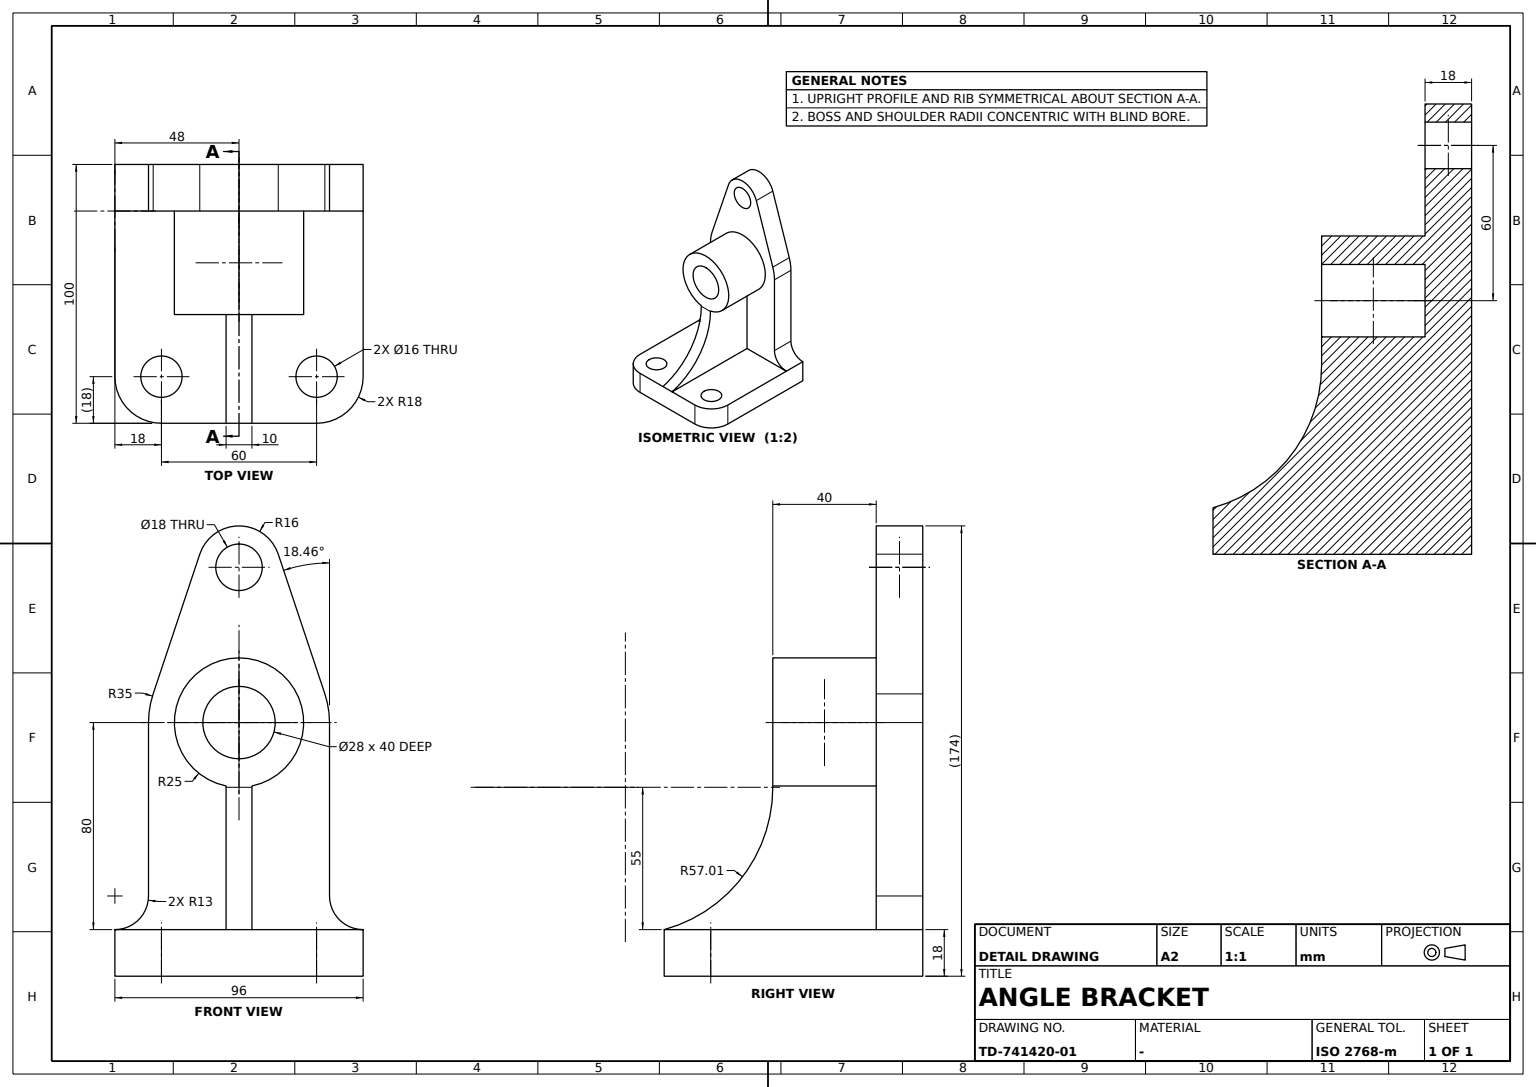
ISO-10303-21;
HEADER;
FILE_DESCRIPTION((''),'2;1');
FILE_NAME('','',(''),(''),'','','');
FILE_SCHEMA(('AUTOMOTIVE_DESIGN'));
ENDSEC;
DATA;
#1=APPLICATION_CONTEXT('');
#2=PRODUCT_CONTEXT('',#1,'mechanical');
#3=PRODUCT('','','',(#2));
#4=PRODUCT_DEFINITION_FORMATION('','',#3);
#5=PRODUCT_DEFINITION_CONTEXT('',#1,'design');
#6=PRODUCT_DEFINITION('','',#4,#5);
#7=PRODUCT_DEFINITION_SHAPE('','',#6);
#8=(LENGTH_UNIT()NAMED_UNIT(*)SI_UNIT(.MILLI.,.METRE.));
#9=(NAMED_UNIT(*)PLANE_ANGLE_UNIT()SI_UNIT($,.RADIAN.));
#10=(NAMED_UNIT(*)SI_UNIT($,.STERADIAN.)SOLID_ANGLE_UNIT());
#11=UNCERTAINTY_MEASURE_WITH_UNIT(LENGTH_MEASURE(0.005),#8,'distance_accuracy_value','');
#12=(GEOMETRIC_REPRESENTATION_CONTEXT(3)GLOBAL_UNCERTAINTY_ASSIGNED_CONTEXT((#11))GLOBAL_UNIT_ASSIGNED_CONTEXT((#8,#9,#10))REPRESENTATION_CONTEXT('',''));
#13=CARTESIAN_POINT('',(-48.,82.,0.));
#14=VERTEX_POINT('',#13);
#15=CARTESIAN_POINT('',(-48.,82.,-18.));
#16=VERTEX_POINT('',#15);
#17=CARTESIAN_POINT('',(-48.,82.,-9.));
#18=DIRECTION('',(0.,0.,1.));
#19=VECTOR('',#18,1000.);
#20=LINE('',#17,#19);
#21=EDGE_CURVE('',#14,#16,#20,.F.);
#22=ORIENTED_EDGE('',*,*,#21,.F.);
#23=CARTESIAN_POINT('',(-30.,100.,0.));
#24=VERTEX_POINT('',#23);
#25=CARTESIAN_POINT('',(-30.,82.,0.));
#26=DIRECTION('',(1.,0.,0.));
#27=AXIS2_PLACEMENT_3D('',#25,#18,#26);
#28=CIRCLE('',#27,18.);
#29=EDGE_CURVE('',#24,#14,#28,.T.);
#30=ORIENTED_EDGE('',*,*,#29,.F.);
#31=CARTESIAN_POINT('',(-30.,100.,-18.));
#32=VERTEX_POINT('',#31);
#33=CARTESIAN_POINT('',(-30.,100.,-9.));
#34=LINE('',#33,#19);
#35=EDGE_CURVE('',#24,#32,#34,.F.);
#36=ORIENTED_EDGE('',*,*,#35,.T.);
#37=CARTESIAN_POINT('',(-30.,82.,-18.));
#38=AXIS2_PLACEMENT_3D('',#37,#18,#26);
#39=CIRCLE('',#38,18.);
#40=EDGE_CURVE('',#32,#16,#39,.T.);
#41=ORIENTED_EDGE('',*,*,#40,.T.);
#42=EDGE_LOOP('',(#22,#30,#36,#41));
#43=FACE_BOUND('',#42,.T.);
#44=CARTESIAN_POINT('',(-30.,82.,-9.));
#45=AXIS2_PLACEMENT_3D('',#44,#18,#26);
#46=CYLINDRICAL_SURFACE('',#45,18.);
#47=ADVANCED_FACE('',(#43),#46,.T.);
#48=CARTESIAN_POINT('',(-35.,0.,80.));
#49=VERTEX_POINT('',#48);
#50=CARTESIAN_POINT('',(-33.198791,0.,91.083333));
#51=VERTEX_POINT('',#50);
#52=CARTESIAN_POINT('',(0.,0.,80.));
#53=DIRECTION('',(0.,-1.,0.));
#54=DIRECTION('',(0.,0.,-1.));
#55=AXIS2_PLACEMENT_3D('',#52,#53,#54);
#56=CIRCLE('',#55,35.);
#57=EDGE_CURVE('',#49,#51,#56,.F.);
#58=ORIENTED_EDGE('',*,*,#57,.T.);
#59=CARTESIAN_POINT('',(-33.198791,18.,91.083333));
#60=VERTEX_POINT('',#59);
#61=CARTESIAN_POINT('',(-33.198791,9.,91.083333));
#62=DIRECTION('',(0.,1.,0.));
#63=VECTOR('',#62,1000.);
#64=LINE('',#61,#63);
#65=EDGE_CURVE('',#51,#60,#64,.T.);
#66=ORIENTED_EDGE('',*,*,#65,.T.);
#67=CARTESIAN_POINT('',(-35.,18.,80.));
#68=VERTEX_POINT('',#67);
#69=CARTESIAN_POINT('',(0.,18.,80.));
#70=AXIS2_PLACEMENT_3D('',#69,#62,#18);
#71=CIRCLE('',#70,35.);
#72=EDGE_CURVE('',#68,#60,#71,.T.);
#73=ORIENTED_EDGE('',*,*,#72,.F.);
#74=CARTESIAN_POINT('',(-35.,9.,80.));
#75=LINE('',#74,#63);
#76=EDGE_CURVE('',#49,#68,#75,.T.);
#77=ORIENTED_EDGE('',*,*,#76,.F.);
#78=EDGE_LOOP('',(#58,#66,#73,#77));
#79=FACE_BOUND('',#78,.T.);
#80=CARTESIAN_POINT('',(0.,9.,80.));
#81=DIRECTION('',(-1.,0.,0.));
#82=AXIS2_PLACEMENT_3D('',#80,#62,#81);
#83=CYLINDRICAL_SURFACE('',#82,35.);
#84=ADVANCED_FACE('',(#79),#83,.T.);
#85=CARTESIAN_POINT('',(35.,18.,80.));
#86=VERTEX_POINT('',#85);
#87=CARTESIAN_POINT('',(35.,18.,13.));
#88=VERTEX_POINT('',#87);
#89=CARTESIAN_POINT('',(35.,18.,0.));
#90=VECTOR('',#54,1000.);
#91=LINE('',#89,#90);
#92=EDGE_CURVE('',#86,#88,#91,.T.);
#93=ORIENTED_EDGE('',*,*,#92,.F.);
#94=CARTESIAN_POINT('',(35.,0.,80.));
#95=VERTEX_POINT('',#94);
#96=CARTESIAN_POINT('',(35.,9.,80.));
#97=LINE('',#96,#63);
#98=EDGE_CURVE('',#95,#86,#97,.T.);
#99=ORIENTED_EDGE('',*,*,#98,.F.);
#100=CARTESIAN_POINT('',(35.,0.,13.));
#101=VERTEX_POINT('',#100);
#102=LINE('',#94,#90);
#103=EDGE_CURVE('',#95,#101,#102,.T.);
#104=ORIENTED_EDGE('',*,*,#103,.T.);
#105=CARTESIAN_POINT('',(35.,50.,13.));
#106=LINE('',#105,#63);
#107=EDGE_CURVE('',#101,#88,#106,.T.);
#108=ORIENTED_EDGE('',*,*,#107,.T.);
#109=EDGE_LOOP('',(#93,#99,#104,#108));
#110=FACE_BOUND('',#109,.T.);
#111=AXIS2_PLACEMENT_3D('',#94,#26,#54);
#112=PLANE('',#111);
#113=ADVANCED_FACE('',(#110),#112,.T.);
#114=CARTESIAN_POINT('',(-5.,100.,0.));
#115=VERTEX_POINT('',#114);
#116=CARTESIAN_POINT('',(5.,100.,0.));
#117=VERTEX_POINT('',#116);
#118=VECTOR('',#26,1000.);
#119=LINE('',#114,#118);
#120=EDGE_CURVE('',#115,#117,#119,.T.);
#121=ORIENTED_EDGE('',*,*,#120,.T.);
#122=CARTESIAN_POINT('',(30.,100.,0.));
#123=VERTEX_POINT('',#122);
#124=LINE('',#23,#118);
#125=EDGE_CURVE('',#117,#123,#124,.T.);
#126=ORIENTED_EDGE('',*,*,#125,.T.);
#127=CARTESIAN_POINT('',(30.,100.,-18.));
#128=VERTEX_POINT('',#127);
#129=CARTESIAN_POINT('',(30.,100.,-9.));
#130=LINE('',#129,#19);
#131=EDGE_CURVE('',#123,#128,#130,.F.);
#132=ORIENTED_EDGE('',*,*,#131,.T.);
#133=LINE('',#31,#118);
#134=EDGE_CURVE('',#32,#128,#133,.T.);
#135=ORIENTED_EDGE('',*,*,#134,.F.);
#136=ORIENTED_EDGE('',*,*,#35,.F.);
#137=EDGE_CURVE('',#24,#115,#124,.T.);
#138=ORIENTED_EDGE('',*,*,#137,.T.);
#139=EDGE_LOOP('',(#121,#126,#132,#135,#136,#138));
#140=FACE_BOUND('',#139,.T.);
#141=AXIS2_PLACEMENT_3D('',#23,#62,#26);
#142=PLANE('',#141);
#143=ADVANCED_FACE('',(#140),#142,.T.);
#144=CARTESIAN_POINT('',(0.,18.,94.));
#145=VERTEX_POINT('',#144);
#146=CIRCLE('',#70,14.);
#147=EDGE_CURVE('',#145,#145,#146,.T.);
#148=ORIENTED_EDGE('',*,*,#147,.F.);
#149=EDGE_LOOP('',(#148));
#150=FACE_BOUND('',#149,.T.);
#151=CARTESIAN_POINT('',(0.,58.,94.));
#152=VERTEX_POINT('',#151);
#153=CARTESIAN_POINT('',(0.,58.,80.));
#154=AXIS2_PLACEMENT_3D('',#153,#62,#18);
#155=CIRCLE('',#154,14.);
#156=EDGE_CURVE('',#152,#152,#155,.T.);
#157=ORIENTED_EDGE('',*,*,#156,.T.);
#158=EDGE_LOOP('',(#157));
#159=FACE_BOUND('',#158,.T.);
#160=CARTESIAN_POINT('',(0.,38.,80.));
#161=AXIS2_PLACEMENT_3D('',#160,#62,#81);
#162=CYLINDRICAL_SURFACE('',#161,14.);
#163=ADVANCED_FACE('',(#150,#159),#162,.F.);
#164=CARTESIAN_POINT('',(0.,0.,131.));
#165=VERTEX_POINT('',#164);
#166=CARTESIAN_POINT('',(0.,0.,140.));
#167=AXIS2_PLACEMENT_3D('',#166,#53,#54);
#168=CIRCLE('',#167,9.);
#169=EDGE_CURVE('',#165,#165,#168,.F.);
#170=ORIENTED_EDGE('',*,*,#169,.T.);
#171=EDGE_LOOP('',(#170));
#172=FACE_BOUND('',#171,.T.);
#173=CARTESIAN_POINT('',(48.,0.,0.));
#174=VERTEX_POINT('',#173);
#175=CARTESIAN_POINT('',(48.,0.,-18.));
#176=VERTEX_POINT('',#175);
#177=LINE('',#173,#90);
#178=EDGE_CURVE('',#174,#176,#177,.T.);
#179=ORIENTED_EDGE('',*,*,#178,.F.);
#180=CARTESIAN_POINT('',(48.,0.,13.));
#181=AXIS2_PLACEMENT_3D('',#180,#53,#54);
#182=CIRCLE('',#181,13.);
#183=EDGE_CURVE('',#101,#174,#182,.T.);
#184=ORIENTED_EDGE('',*,*,#183,.F.);
#185=ORIENTED_EDGE('',*,*,#103,.F.);
#186=CARTESIAN_POINT('',(33.198791,0.,91.083333));
#187=VERTEX_POINT('',#186);
#188=EDGE_CURVE('',#187,#95,#56,.F.);
#189=ORIENTED_EDGE('',*,*,#188,.F.);
#190=CARTESIAN_POINT('',(15.17659,0.,145.066667));
#191=VERTEX_POINT('',#190);
#192=DIRECTION('',(0.316666667,0.,-0.948536885));
#193=VECTOR('',#192,1000.);
#194=LINE('',#190,#193);
#195=EDGE_CURVE('',#191,#187,#194,.T.);
#196=ORIENTED_EDGE('',*,*,#195,.F.);
#197=CARTESIAN_POINT('',(-15.17659,0.,145.066667));
#198=VERTEX_POINT('',#197);
#199=CIRCLE('',#167,16.);
#200=EDGE_CURVE('',#198,#191,#199,.F.);
#201=ORIENTED_EDGE('',*,*,#200,.F.);
#202=DIRECTION('',(-0.316666667,0.,-0.948536885));
#203=VECTOR('',#202,1000.);
#204=LINE('',#197,#203);
#205=EDGE_CURVE('',#198,#51,#204,.T.);
#206=ORIENTED_EDGE('',*,*,#205,.T.);
#207=ORIENTED_EDGE('',*,*,#57,.F.);
#208=CARTESIAN_POINT('',(-35.,0.,13.));
#209=VERTEX_POINT('',#208);
#210=LINE('',#48,#90);
#211=EDGE_CURVE('',#49,#209,#210,.T.);
#212=ORIENTED_EDGE('',*,*,#211,.T.);
#213=CARTESIAN_POINT('',(-48.,0.,0.));
#214=VERTEX_POINT('',#213);
#215=CARTESIAN_POINT('',(-48.,0.,13.));
#216=AXIS2_PLACEMENT_3D('',#215,#53,#54);
#217=CIRCLE('',#216,13.);
#218=EDGE_CURVE('',#214,#209,#217,.T.);
#219=ORIENTED_EDGE('',*,*,#218,.F.);
#220=CARTESIAN_POINT('',(-48.,0.,-18.));
#221=VERTEX_POINT('',#220);
#222=LINE('',#213,#90);
#223=EDGE_CURVE('',#214,#221,#222,.T.);
#224=ORIENTED_EDGE('',*,*,#223,.T.);
#225=VECTOR('',#81,1000.);
#226=LINE('',#175,#225);
#227=EDGE_CURVE('',#176,#221,#226,.T.);
#228=ORIENTED_EDGE('',*,*,#227,.F.);
#229=EDGE_LOOP('',(#179,#184,#185,#189,#196,#201,#206,#207,#212,#219,#224,#228));
#230=FACE_BOUND('',#229,.T.);
#231=AXIS2_PLACEMENT_3D('',#173,#53,#81);
#232=PLANE('',#231);
#233=ADVANCED_FACE('',(#172,#230),#232,.T.);
#234=CARTESIAN_POINT('',(-35.,18.,13.));
#235=VERTEX_POINT('',#234);
#236=CARTESIAN_POINT('',(-48.,18.,0.));
#237=VERTEX_POINT('',#236);
#238=CARTESIAN_POINT('',(-48.,18.,13.));
#239=AXIS2_PLACEMENT_3D('',#238,#62,#18);
#240=CIRCLE('',#239,13.);
#241=EDGE_CURVE('',#235,#237,#240,.T.);
#242=ORIENTED_EDGE('',*,*,#241,.T.);
#243=LINE('',#236,#63);
#244=EDGE_CURVE('',#237,#214,#243,.F.);
#245=ORIENTED_EDGE('',*,*,#244,.T.);
#246=ORIENTED_EDGE('',*,*,#218,.T.);
#247=CARTESIAN_POINT('',(-35.,50.,13.));
#248=LINE('',#247,#63);
#249=EDGE_CURVE('',#209,#235,#248,.T.);
#250=ORIENTED_EDGE('',*,*,#249,.T.);
#251=EDGE_LOOP('',(#242,#245,#246,#250));
#252=FACE_BOUND('',#251,.T.);
#253=CARTESIAN_POINT('',(-48.,50.,13.));
#254=AXIS2_PLACEMENT_3D('',#253,#62,#26);
#255=CYLINDRICAL_SURFACE('',#254,13.);
#256=ADVANCED_FACE('',(#252),#255,.F.);
#257=CARTESIAN_POINT('',(-5.,58.,55.505103));
#258=VERTEX_POINT('',#257);
#259=CARTESIAN_POINT('',(5.,58.,55.505103));
#260=VERTEX_POINT('',#259);
#261=CIRCLE('',#154,25.);
#262=EDGE_CURVE('',#258,#260,#261,.T.);
#263=ORIENTED_EDGE('',*,*,#262,.F.);
#264=CARTESIAN_POINT('',(-5.,18.,55.505103));
#265=VERTEX_POINT('',#264);
#266=LINE('',#264,#63);
#267=EDGE_CURVE('',#265,#258,#266,.T.);
#268=ORIENTED_EDGE('',*,*,#267,.F.);
#269=CARTESIAN_POINT('',(5.,18.,55.505103));
#270=VERTEX_POINT('',#269);
#271=CIRCLE('',#70,25.);
#272=EDGE_CURVE('',#265,#270,#271,.T.);
#273=ORIENTED_EDGE('',*,*,#272,.T.);
#274=LINE('',#269,#63);
#275=EDGE_CURVE('',#270,#260,#274,.T.);
#276=ORIENTED_EDGE('',*,*,#275,.T.);
#277=EDGE_LOOP('',(#263,#268,#273,#276));
#278=FACE_BOUND('',#277,.T.);
#279=CYLINDRICAL_SURFACE('',#161,25.);
#280=ADVANCED_FACE('',(#278),#279,.T.);
#281=ORIENTED_EDGE('',*,*,#205,.F.);
#282=CARTESIAN_POINT('',(-15.17659,18.,145.066667));
#283=VERTEX_POINT('',#282);
#284=CARTESIAN_POINT('',(-15.17659,9.,145.066667));
#285=LINE('',#284,#63);
#286=EDGE_CURVE('',#198,#283,#285,.T.);
#287=ORIENTED_EDGE('',*,*,#286,.T.);
#288=CARTESIAN_POINT('',(-57.228392,18.,19.105556));
#289=LINE('',#288,#203);
#290=EDGE_CURVE('',#283,#60,#289,.T.);
#291=ORIENTED_EDGE('',*,*,#290,.T.);
#292=ORIENTED_EDGE('',*,*,#65,.F.);
#293=EDGE_LOOP('',(#281,#287,#291,#292));
#294=FACE_BOUND('',#293,.T.);
#295=DIRECTION('',(0.948536885,0.,-0.316666667));
#296=AXIS2_PLACEMENT_3D('',#197,#295,#202);
#297=PLANE('',#296);
#298=ADVANCED_FACE('',(#294),#297,.F.);
#299=CARTESIAN_POINT('',(-5.,58.,55.));
#300=VERTEX_POINT('',#299);
#301=CARTESIAN_POINT('',(-5.,115.011905,55.));
#302=AXIS2_PLACEMENT_3D('',#301,#26,#54);
#303=CIRCLE('',#302,57.011905);
#304=EDGE_CURVE('',#300,#115,#303,.T.);
#305=ORIENTED_EDGE('',*,*,#304,.F.);
#306=CARTESIAN_POINT('',(5.,58.,55.));
#307=VERTEX_POINT('',#306);
#308=CARTESIAN_POINT('',(0.,58.,55.));
#309=LINE('',#308,#118);
#310=EDGE_CURVE('',#300,#307,#309,.T.);
#311=ORIENTED_EDGE('',*,*,#310,.T.);
#312=CARTESIAN_POINT('',(5.,115.011905,55.));
#313=AXIS2_PLACEMENT_3D('',#312,#26,#54);
#314=CIRCLE('',#313,57.011905);
#315=EDGE_CURVE('',#307,#117,#314,.T.);
#316=ORIENTED_EDGE('',*,*,#315,.T.);
#317=ORIENTED_EDGE('',*,*,#120,.F.);
#318=EDGE_LOOP('',(#305,#311,#316,#317));
#319=FACE_BOUND('',#318,.T.);
#320=CARTESIAN_POINT('',(0.,115.011905,55.));
#321=AXIS2_PLACEMENT_3D('',#320,#26,#62);
#322=CYLINDRICAL_SURFACE('',#321,57.011905);
#323=ADVANCED_FACE('',(#319),#322,.F.);
#324=ORIENTED_EDGE('',*,*,#147,.T.);
#325=EDGE_LOOP('',(#324));
#326=FACE_BOUND('',#325,.T.);
#327=CARTESIAN_POINT('',(0.,18.,0.));
#328=AXIS2_PLACEMENT_3D('',#327,#62,#81);
#329=PLANE('',#328);
#330=ADVANCED_FACE('',(#326),#329,.T.);
#331=CARTESIAN_POINT('',(48.,18.,0.));
#332=VERTEX_POINT('',#331);
#333=LINE('',#173,#63);
#334=EDGE_CURVE('',#174,#332,#333,.T.);
#335=ORIENTED_EDGE('',*,*,#334,.F.);
#336=ORIENTED_EDGE('',*,*,#178,.T.);
#337=CARTESIAN_POINT('',(48.,82.,-18.));
#338=VERTEX_POINT('',#337);
#339=LINE('',#175,#63);
#340=EDGE_CURVE('',#176,#338,#339,.T.);
#341=ORIENTED_EDGE('',*,*,#340,.T.);
#342=CARTESIAN_POINT('',(48.,82.,0.));
#343=VERTEX_POINT('',#342);
#344=CARTESIAN_POINT('',(48.,82.,-9.));
#345=LINE('',#344,#19);
#346=EDGE_CURVE('',#343,#338,#345,.F.);
#347=ORIENTED_EDGE('',*,*,#346,.F.);
#348=EDGE_CURVE('',#332,#343,#333,.T.);
#349=ORIENTED_EDGE('',*,*,#348,.F.);
#350=EDGE_LOOP('',(#335,#336,#341,#347,#349));
#351=FACE_BOUND('',#350,.T.);
#352=AXIS2_PLACEMENT_3D('',#173,#81,#62);
#353=PLANE('',#352);
#354=ADVANCED_FACE('',(#351),#353,.F.);
#355=CARTESIAN_POINT('',(38.,82.,0.));
#356=VERTEX_POINT('',#355);
#357=CARTESIAN_POINT('',(30.,82.,0.));
#358=AXIS2_PLACEMENT_3D('',#357,#18,#26);
#359=CIRCLE('',#358,8.);
#360=EDGE_CURVE('',#356,#356,#359,.T.);
#361=ORIENTED_EDGE('',*,*,#360,.F.);
#362=EDGE_LOOP('',(#361));
#363=FACE_BOUND('',#362,.T.);
#364=CIRCLE('',#358,18.);
#365=EDGE_CURVE('',#343,#123,#364,.T.);
#366=ORIENTED_EDGE('',*,*,#365,.T.);
#367=ORIENTED_EDGE('',*,*,#125,.F.);
#368=CARTESIAN_POINT('',(5.,18.,0.));
#369=VERTEX_POINT('',#368);
#370=CARTESIAN_POINT('',(5.,0.,0.));
#371=VECTOR('',#53,1000.);
#372=LINE('',#370,#371);
#373=EDGE_CURVE('',#117,#369,#372,.T.);
#374=ORIENTED_EDGE('',*,*,#373,.T.);
#375=LINE('',#327,#118);
#376=EDGE_CURVE('',#369,#332,#375,.T.);
#377=ORIENTED_EDGE('',*,*,#376,.T.);
#378=ORIENTED_EDGE('',*,*,#348,.T.);
#379=EDGE_LOOP('',(#366,#367,#374,#377,#378));
#380=FACE_BOUND('',#379,.T.);
#381=CARTESIAN_POINT('',(0.,0.,0.));
#382=AXIS2_PLACEMENT_3D('',#381,#18,#26);
#383=PLANE('',#382);
#384=ADVANCED_FACE('',(#363,#380),#383,.T.);
#385=CARTESIAN_POINT('',(38.,82.,-18.));
#386=VERTEX_POINT('',#385);
#387=CARTESIAN_POINT('',(30.,82.,-18.));
#388=AXIS2_PLACEMENT_3D('',#387,#18,#26);
#389=CIRCLE('',#388,8.);
#390=EDGE_CURVE('',#386,#386,#389,.T.);
#391=ORIENTED_EDGE('',*,*,#390,.F.);
#392=EDGE_LOOP('',(#391));
#393=FACE_BOUND('',#392,.T.);
#394=ORIENTED_EDGE('',*,*,#360,.T.);
#395=EDGE_LOOP('',(#394));
#396=FACE_BOUND('',#395,.T.);
#397=CARTESIAN_POINT('',(30.,82.,-9.));
#398=AXIS2_PLACEMENT_3D('',#397,#18,#26);
#399=CYLINDRICAL_SURFACE('',#398,8.);
#400=ADVANCED_FACE('',(#393,#396),#399,.F.);
#401=CARTESIAN_POINT('',(15.17659,18.,145.066667));
#402=VERTEX_POINT('',#401);
#403=CARTESIAN_POINT('',(0.,18.,140.));
#404=AXIS2_PLACEMENT_3D('',#403,#62,#18);
#405=CIRCLE('',#404,16.);
#406=EDGE_CURVE('',#283,#402,#405,.T.);
#407=ORIENTED_EDGE('',*,*,#406,.F.);
#408=ORIENTED_EDGE('',*,*,#286,.F.);
#409=ORIENTED_EDGE('',*,*,#200,.T.);
#410=CARTESIAN_POINT('',(15.17659,9.,145.066667));
#411=LINE('',#410,#63);
#412=EDGE_CURVE('',#191,#402,#411,.T.);
#413=ORIENTED_EDGE('',*,*,#412,.T.);
#414=EDGE_LOOP('',(#407,#408,#409,#413));
#415=FACE_BOUND('',#414,.T.);
#416=CARTESIAN_POINT('',(0.,9.,140.));
#417=AXIS2_PLACEMENT_3D('',#416,#62,#81);
#418=CYLINDRICAL_SURFACE('',#417,16.);
#419=ADVANCED_FACE('',(#415),#418,.T.);
#420=ORIENTED_EDGE('',*,*,#249,.F.);
#421=ORIENTED_EDGE('',*,*,#211,.F.);
#422=ORIENTED_EDGE('',*,*,#76,.T.);
#423=CARTESIAN_POINT('',(-35.,18.,0.));
#424=LINE('',#423,#90);
#425=EDGE_CURVE('',#68,#235,#424,.T.);
#426=ORIENTED_EDGE('',*,*,#425,.T.);
#427=EDGE_LOOP('',(#420,#421,#422,#426));
#428=FACE_BOUND('',#427,.T.);
#429=AXIS2_PLACEMENT_3D('',#48,#26,#54);
#430=PLANE('',#429);
#431=ADVANCED_FACE('',(#428),#430,.F.);
#432=LINE('',#15,#371);
#433=EDGE_CURVE('',#16,#221,#432,.T.);
#434=ORIENTED_EDGE('',*,*,#433,.T.);
#435=ORIENTED_EDGE('',*,*,#223,.F.);
#436=ORIENTED_EDGE('',*,*,#244,.F.);
#437=LINE('',#13,#371);
#438=EDGE_CURVE('',#14,#237,#437,.T.);
#439=ORIENTED_EDGE('',*,*,#438,.F.);
#440=ORIENTED_EDGE('',*,*,#21,.T.);
#441=EDGE_LOOP('',(#434,#435,#436,#439,#440));
#442=FACE_BOUND('',#441,.T.);
#443=AXIS2_PLACEMENT_3D('',#13,#26,#53);
#444=PLANE('',#443);
#445=ADVANCED_FACE('',(#442),#444,.F.);
#446=CARTESIAN_POINT('',(-22.,82.,0.));
#447=VERTEX_POINT('',#446);
#448=CIRCLE('',#27,8.);
#449=EDGE_CURVE('',#447,#447,#448,.T.);
#450=ORIENTED_EDGE('',*,*,#449,.F.);
#451=EDGE_LOOP('',(#450));
#452=FACE_BOUND('',#451,.T.);
#453=ORIENTED_EDGE('',*,*,#438,.T.);
#454=CARTESIAN_POINT('',(-5.,18.,0.));
#455=VERTEX_POINT('',#454);
#456=EDGE_CURVE('',#237,#455,#375,.T.);
#457=ORIENTED_EDGE('',*,*,#456,.T.);
#458=CARTESIAN_POINT('',(-5.,0.,0.));
#459=LINE('',#458,#371);
#460=EDGE_CURVE('',#115,#455,#459,.T.);
#461=ORIENTED_EDGE('',*,*,#460,.F.);
#462=ORIENTED_EDGE('',*,*,#137,.F.);
#463=ORIENTED_EDGE('',*,*,#29,.T.);
#464=EDGE_LOOP('',(#453,#457,#461,#462,#463));
#465=FACE_BOUND('',#464,.T.);
#466=ADVANCED_FACE('',(#452,#465),#383,.T.);
#467=ORIENTED_EDGE('',*,*,#376,.F.);
#468=LINE('',#368,#90);
#469=EDGE_CURVE('',#270,#369,#468,.T.);
#470=ORIENTED_EDGE('',*,*,#469,.F.);
#471=ORIENTED_EDGE('',*,*,#272,.F.);
#472=LINE('',#454,#90);
#473=EDGE_CURVE('',#265,#455,#472,.T.);
#474=ORIENTED_EDGE('',*,*,#473,.T.);
#475=ORIENTED_EDGE('',*,*,#456,.F.);
#476=ORIENTED_EDGE('',*,*,#241,.F.);
#477=ORIENTED_EDGE('',*,*,#425,.F.);
#478=ORIENTED_EDGE('',*,*,#72,.T.);
#479=ORIENTED_EDGE('',*,*,#290,.F.);
#480=ORIENTED_EDGE('',*,*,#406,.T.);
#481=CARTESIAN_POINT('',(33.198791,18.,91.083333));
#482=VERTEX_POINT('',#481);
#483=CARTESIAN_POINT('',(57.228392,18.,19.105556));
#484=LINE('',#483,#193);
#485=EDGE_CURVE('',#402,#482,#484,.T.);
#486=ORIENTED_EDGE('',*,*,#485,.T.);
#487=EDGE_CURVE('',#482,#86,#71,.T.);
#488=ORIENTED_EDGE('',*,*,#487,.T.);
#489=ORIENTED_EDGE('',*,*,#92,.T.);
#490=CARTESIAN_POINT('',(48.,18.,13.));
#491=AXIS2_PLACEMENT_3D('',#490,#62,#18);
#492=CIRCLE('',#491,13.);
#493=EDGE_CURVE('',#332,#88,#492,.T.);
#494=ORIENTED_EDGE('',*,*,#493,.F.);
#495=EDGE_LOOP('',(#467,#470,#471,#474,#475,#476,#477,#478,#479,#480,#486,#488,#489,#494));
#496=FACE_BOUND('',#495,.T.);
#497=CARTESIAN_POINT('',(0.,18.,149.));
#498=VERTEX_POINT('',#497);
#499=CIRCLE('',#404,9.);
#500=EDGE_CURVE('',#498,#498,#499,.T.);
#501=ORIENTED_EDGE('',*,*,#500,.F.);
#502=EDGE_LOOP('',(#501));
#503=FACE_BOUND('',#502,.T.);
#504=ADVANCED_FACE('',(#496,#503),#329,.T.);
#505=ORIENTED_EDGE('',*,*,#365,.F.);
#506=ORIENTED_EDGE('',*,*,#346,.T.);
#507=CIRCLE('',#388,18.);
#508=EDGE_CURVE('',#338,#128,#507,.T.);
#509=ORIENTED_EDGE('',*,*,#508,.T.);
#510=ORIENTED_EDGE('',*,*,#131,.F.);
#511=EDGE_LOOP('',(#505,#506,#509,#510));
#512=FACE_BOUND('',#511,.T.);
#513=CYLINDRICAL_SURFACE('',#398,18.);
#514=ADVANCED_FACE('',(#512),#513,.T.);
#515=ORIENTED_EDGE('',*,*,#390,.T.);
#516=EDGE_LOOP('',(#515));
#517=FACE_BOUND('',#516,.T.);
#518=CARTESIAN_POINT('',(-22.,82.,-18.));
#519=VERTEX_POINT('',#518);
#520=CIRCLE('',#38,8.);
#521=EDGE_CURVE('',#519,#519,#520,.T.);
#522=ORIENTED_EDGE('',*,*,#521,.T.);
#523=EDGE_LOOP('',(#522));
#524=FACE_BOUND('',#523,.T.);
#525=ORIENTED_EDGE('',*,*,#433,.F.);
#526=ORIENTED_EDGE('',*,*,#40,.F.);
#527=ORIENTED_EDGE('',*,*,#134,.T.);
#528=ORIENTED_EDGE('',*,*,#508,.F.);
#529=ORIENTED_EDGE('',*,*,#340,.F.);
#530=ORIENTED_EDGE('',*,*,#227,.T.);
#531=EDGE_LOOP('',(#525,#526,#527,#528,#529,#530));
#532=FACE_BOUND('',#531,.T.);
#533=CARTESIAN_POINT('',(0.,0.,-18.));
#534=AXIS2_PLACEMENT_3D('',#533,#18,#26);
#535=PLANE('',#534);
#536=ADVANCED_FACE('',(#517,#524,#532),#535,.F.);
#537=ORIENTED_EDGE('',*,*,#188,.T.);
#538=ORIENTED_EDGE('',*,*,#98,.T.);
#539=ORIENTED_EDGE('',*,*,#487,.F.);
#540=CARTESIAN_POINT('',(33.198791,9.,91.083333));
#541=LINE('',#540,#63);
#542=EDGE_CURVE('',#187,#482,#541,.T.);
#543=ORIENTED_EDGE('',*,*,#542,.F.);
#544=EDGE_LOOP('',(#537,#538,#539,#543));
#545=FACE_BOUND('',#544,.T.);
#546=ADVANCED_FACE('',(#545),#83,.T.);
#547=ORIENTED_EDGE('',*,*,#473,.F.);
#548=ORIENTED_EDGE('',*,*,#267,.T.);
#549=CARTESIAN_POINT('',(-5.,58.,0.));
#550=LINE('',#549,#19);
#551=EDGE_CURVE('',#300,#258,#550,.T.);
#552=ORIENTED_EDGE('',*,*,#551,.F.);
#553=ORIENTED_EDGE('',*,*,#304,.T.);
#554=ORIENTED_EDGE('',*,*,#460,.T.);
#555=EDGE_LOOP('',(#547,#548,#552,#553,#554));
#556=FACE_BOUND('',#555,.T.);
#557=AXIS2_PLACEMENT_3D('',#458,#26,#62);
#558=PLANE('',#557);
#559=ADVANCED_FACE('',(#556),#558,.F.);
#560=ORIENTED_EDGE('',*,*,#449,.T.);
#561=EDGE_LOOP('',(#560));
#562=FACE_BOUND('',#561,.T.);
#563=ORIENTED_EDGE('',*,*,#521,.F.);
#564=EDGE_LOOP('',(#563));
#565=FACE_BOUND('',#564,.T.);
#566=CYLINDRICAL_SURFACE('',#45,8.);
#567=ADVANCED_FACE('',(#562,#565),#566,.F.);
#568=ORIENTED_EDGE('',*,*,#183,.T.);
#569=ORIENTED_EDGE('',*,*,#334,.T.);
#570=ORIENTED_EDGE('',*,*,#493,.T.);
#571=ORIENTED_EDGE('',*,*,#107,.F.);
#572=EDGE_LOOP('',(#568,#569,#570,#571));
#573=FACE_BOUND('',#572,.T.);
#574=CARTESIAN_POINT('',(48.,50.,13.));
#575=AXIS2_PLACEMENT_3D('',#574,#62,#54);
#576=CYLINDRICAL_SURFACE('',#575,13.);
#577=ADVANCED_FACE('',(#573),#576,.F.);
#578=ORIENTED_EDGE('',*,*,#195,.T.);
#579=ORIENTED_EDGE('',*,*,#542,.T.);
#580=ORIENTED_EDGE('',*,*,#485,.F.);
#581=ORIENTED_EDGE('',*,*,#412,.F.);
#582=EDGE_LOOP('',(#578,#579,#580,#581));
#583=FACE_BOUND('',#582,.T.);
#584=DIRECTION('',(0.948536885,0.,0.316666667));
#585=AXIS2_PLACEMENT_3D('',#190,#584,#192);
#586=PLANE('',#585);
#587=ADVANCED_FACE('',(#583),#586,.T.);
#588=ORIENTED_EDGE('',*,*,#156,.F.);
#589=EDGE_LOOP('',(#588));
#590=FACE_BOUND('',#589,.T.);
#591=CARTESIAN_POINT('',(5.,58.,0.));
#592=LINE('',#591,#19);
#593=EDGE_CURVE('',#307,#260,#592,.T.);
#594=ORIENTED_EDGE('',*,*,#593,.F.);
#595=ORIENTED_EDGE('',*,*,#310,.F.);
#596=ORIENTED_EDGE('',*,*,#551,.T.);
#597=ORIENTED_EDGE('',*,*,#262,.T.);
#598=EDGE_LOOP('',(#594,#595,#596,#597));
#599=FACE_BOUND('',#598,.T.);
#600=CARTESIAN_POINT('',(0.,58.,0.));
#601=AXIS2_PLACEMENT_3D('',#600,#62,#81);
#602=PLANE('',#601);
#603=ADVANCED_FACE('',(#590,#599),#602,.T.);
#604=ORIENTED_EDGE('',*,*,#500,.T.);
#605=EDGE_LOOP('',(#604));
#606=FACE_BOUND('',#605,.T.);
#607=ORIENTED_EDGE('',*,*,#169,.F.);
#608=EDGE_LOOP('',(#607));
#609=FACE_BOUND('',#608,.T.);
#610=CYLINDRICAL_SURFACE('',#417,9.);
#611=ADVANCED_FACE('',(#606,#609),#610,.F.);
#612=ORIENTED_EDGE('',*,*,#275,.F.);
#613=ORIENTED_EDGE('',*,*,#469,.T.);
#614=ORIENTED_EDGE('',*,*,#373,.F.);
#615=ORIENTED_EDGE('',*,*,#315,.F.);
#616=ORIENTED_EDGE('',*,*,#593,.T.);
#617=EDGE_LOOP('',(#612,#613,#614,#615,#616));
#618=FACE_BOUND('',#617,.T.);
#619=AXIS2_PLACEMENT_3D('',#370,#26,#62);
#620=PLANE('',#619);
#621=ADVANCED_FACE('',(#618),#620,.T.);
#622=CLOSED_SHELL('',(#47,#84,#113,#143,#163,#233,#256,#280,#298,#323,#330,#354,#384,#400,#419,#431,#445,#466,#504,#514,#536,#546,#559,#567,#577,#587,#603,#611,#621));
#623=MANIFOLD_SOLID_BREP('',#622);
#624=ADVANCED_BREP_SHAPE_REPRESENTATION('',(#623),#12);
#625=SHAPE_DEFINITION_REPRESENTATION(#7,#624);
ENDSEC;
END-ISO-10303-21;
